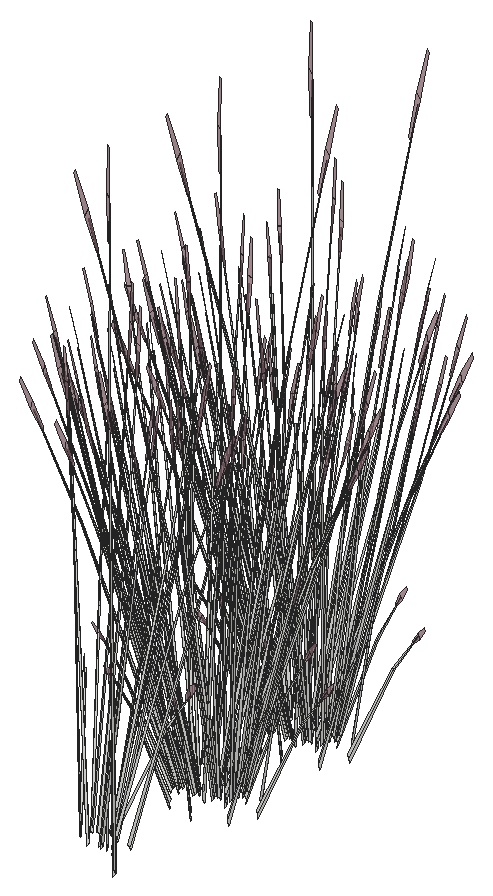
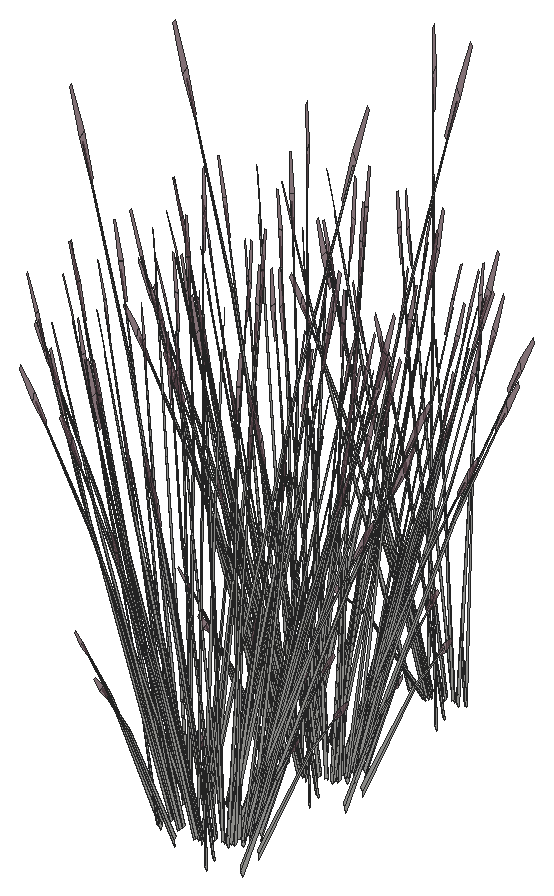
# SketchUp Ruby script. Lengths in inches.
U = 1.inch
M = Sketchup.active_model
def pt(a) = Geom::Point3d.new(a.map { |v| v * U })
def face(e, loops, mat)
  f = e.add_face(loops[0].map { |a| pt(a) })
  loops[1..].each { |l| e.add_face(l.map { |a| pt(a) }).erase! }
  f.material = f.back_material = mat if mat
  f
end
# faces: each face lists its corners as indices into pts; further lists are holes
def faces(e, pts, list, mat = nil) = list.each { |f| face(e, (f[0].is_a?(Array) ? f : [f]).map { |l| l.map { |i| pts[i] } }, mat) }
# xy, xz, yz: faces in a plane at the given z, y or x. An outline is a flat list of corners, or four numbers for a rectangle; further outlines are holes
def ring(l) = l.size == 4 ? [[l[0], l[1]], [l[2], l[1]], [l[2], l[3]], [l[0], l[3]]] : l.each_slice(2).to_a
def flat(e, list, mat, &to3) = list.each { |f| face(e, (f[0].is_a?(Array) ? f : [f]).map { |l| ring(l).map { |u, v| to3.(u, v) } }, mat) }
def xy(e, z, list, mat = nil) = flat(e, list, mat) { |x, y| [x, y, z] }
def xz(e, y, list, mat = nil) = flat(e, list, mat) { |x, z| [x, y, z] }
def yz(e, x, list, mat = nil) = flat(e, list, mat) { |y, z| [x, y, z] }
def lines(e, pts, list) = list.each { |a, b| e.add_line(pt(pts[a]), pt(pts[b])) }
# prism: a flat outline (further loops are holes) pulled along v
def prism(e, loops, v, mat = nil)
  f = face(e, loops, mat); d = Geom::Vector3d.new(v.map { |x| x * U })
  f.pushpull(f.normal.samedirection?(d) ? d.length : -d.length)
end
def box(e, o, s, mat = nil) = prism(e, [[o, [o[0] + s[0], o[1], o[2]], [o[0] + s[0], o[1] + s[1], o[2]], [o[0], o[1] + s[1], o[2]]]], [0, 0, s[2]], mat)
def at(x, y, z, deg = 0) = Geom::Transformation.translation(pt([x, y, z])) * Geom::Transformation.rotation(ORIGIN, Z_AXIS, deg.degrees)
def axes(o, x, y, z) = Geom::Transformation.new([*x, 0, *y, 0, *z, 0, *pt(o).to_a, 1])
def part(name) = M.definitions.add(name)
# library, detail: a bought-in or finely detailed component or shape, given as its bounding box
def library(name, o, s) = part(name).tap { |d| box(d.entities, o, s) }
def detail(e, o, s) = box(e.add_group.entities, o, s)
def put(e, d, t, mat = nil) = e.add_instance(d, t).tap { |i| i.material = mat if mat }
def group(e, t, mat = nil) = e.add_group.tap { |g| g.transformation = t; g.material = mat if mat }.entities
root = M.entities
M.materials.add("LightPink_Translucent").color = [144, 107, 117]
M.materials["LightPink_Translucent"].alpha = 0.75
c1 = part("blade")
p = [[2.15,0.21,22],[0,0.17,0],[0.09,0.45,0],[2.18,0.31,22],[2.29,0.31,22],[0.38,0.45,0],
  [2.48,0.24,33],[2.49,0.24,33],[2.48,0.22,33]]
faces(c1.entities,p,[[0,1,2,3],[4,5,2,3],[6,3,4,7],[8,0,3,6]])
c2 = part("seeds")
p = [[0.3,-0.1,1.38],[-0.01,-0.03,1.59],[-0.01,-0.03,0.03],[0.14,-0.07,-0.07],[0.29,-0.03,3],[0.15,0.01,3.11]]
faces(c2.entities,p,[[0,1,2,3],[1,0,4,5]],"LightPink_Translucent")
c3 = part("blade with seeds")
put(c3.entities,c1,at(0,0,0))
put(c3.entities,c2,axes([2.4,0.25,30.99],[1.5799,-0.05474,1.17369],[-0.12525,1.92788,0.29478],[-0.07173,-0.02425,1.56792]))
put(root,c3,axes([331.86,478.88,52.14],[0.12971,0.3568,-0.45151],[-0.49122,0.06241,-0.34973],[-0.14077,0.09583,0.86392]))
put(root,c3,axes([334.74,478.15,50.51],[-0.01379,-0.36791,1.24828],[0.62424,0.09537,0.52853],[-0.14764,0.20132,1.17828]))
put(root,c3,axes([334.79,479.57,52.14],[0.49824,-0.09289,-0.45151],[0.08716,0.35177,-0.34973],[0.13382,0.10081,0.86392]))
put(root,c3,axes([332.16,478.82,51.43],[0.09401,-0.13431,1.51428],[0.3944,0.27795,0.12244],[-0.17792,0.17323,0.64734]))
put(root,c3,axes([332.27,479.58,52],[-0.34164,0.20573,-0.31292],[-0.3234,-0.23491,0.40398],[-0.04921,0.11936,0.77298]))
put(root,c3,axes([331.09,479.52,52.17],[-0.01255,0.07733,1.54581],[0.35618,0.269,-0.24447],[-0.09325,0.12721,0.12397]))
put(root,c3,axes([333.25,479.75,52.45],[0.49409,-0.18193,-0.10745],[0.24281,0.32289,-0.59638],[0.06519,0.13607,0.90619]))
put(root,c3,axes([332.48,480.38,50.44],[-0.01307,-0.23234,1.01491],[0.32652,0.16572,0.74569],[-0.06422,0.11074,0.22354]))
put(root,c3,axes([332.61,479.48,52.42],[0.36145,0.26255,-0.50118],[-0.38183,0.22994,-0.3882],[-0.055,0.1334,0.95895]))
put(root,c3,axes([333.68,479.74,52.14],[0.49634,0.09796,-0.45151],[-0.17013,0.33585,-0.34973],[0.04551,0.13522,0.86392]))
put(root,c3,axes([333.96,479.04,51.43],[-0.11542,-0.12546,1.51428],[0.53333,-0.10562,0.12244],[0.12054,0.19696,0.64734]))
put(root,c3,axes([333.45,479.94,52],[-0.15222,0.30049,-0.31292],[-0.44409,-0.08764,0.40398],[0.04072,0.12098,0.77298]))
put(root,c3,axes([332.49,479.36,52.72],[-0.01314,0.36145,-0.69681],[-0.55324,-0.02428,0.08409],[-0.05838,0.15313,0.9857]))
put(root,c3,axes([333.02,479.11,51.43],[-0.01236,-0.14998,1.51428],[0.53562,0.09949,0.12244],[-0.03313,0.21373,0.64734]))
put(root,c3,axes([333.5,479.67,52.4],[0.24099,0.31773,-0.62776],[-0.49607,0.17707,0.07576],[0.05635,0.15352,0.88802]))
put(root,c3,axes([333.14,480.48,52.17],[0.064,0.06292,1.54581],[0.51651,0.02472,-0.24447],[0.05194,0.13877,0.12397]))
put(root,c3,axes([332.31,479.87,50.97],[0.01109,-0.20172,1.3638],[0.49896,0.10655,0.18846],[-0.04323,0.21498,0.64398]))
put(root,c3,axes([332.69,487.29,51.43],[0.11542,0.12546,1.51428],[-0.53333,0.10562,0.12244],[-0.12054,-0.19696,0.64734]))
put(root,c3,axes([334.11,487.38,52.4],[-0.24099,-0.31773,-0.62776],[0.49607,-0.17707,0.07576],[-0.05635,-0.15352,0.88802]))
put(root,c3,axes([335.12,487.69,52.4],[0.01314,-0.36145,-0.62776],[0.55324,0.02428,0.07576],[0.05838,-0.15313,0.88802]))
put(root,c3,axes([334.16,487.11,52],[0.15222,-0.30049,-0.31292],[0.44409,0.08764,0.40398],[-0.04072,-0.12098,0.77298]))
put(root,c3,axes([334.5,487.51,51.43],[-0.09401,0.13431,1.51428],[-0.3944,-0.27795,0.12244],[0.17792,-0.17323,0.64734]))
put(root,c3,axes([333.93,487.32,52.14],[-0.49634,-0.09796,-0.45151],[0.17013,-0.33585,-0.34973],[-0.04551,-0.13522,0.86392]))
put(root,c3,axes([334.24,486.48,50.44],[0.06477,0.22786,1.01491],[-0.35932,-0.1262,0.74569],[0.03867,-0.11667,0.22354]))
put(root,c3,axes([335.01,487.57,52.14],[-0.36145,-0.26255,-0.45151],[0.38183,-0.22994,-0.34973],[0.055,-0.1334,0.86392]))
put(root,c3,axes([334.36,487.3,52.45],[-0.49409,0.18193,-0.10745],[-0.24281,-0.32289,-0.59638],[-0.06519,-0.13607,0.90619]))
put(root,c3,axes([335.38,487.71,52.45],[-0.55492,-0.01936,-0.10745],[0.01517,-0.36657,-0.59638],[0.03855,-0.14118,0.90619]))
put(root,c3,axes([335.35,487.47,52],[0.34164,-0.20573,-0.31292],[0.3234,0.23491,0.40398],[0.04921,-0.11936,0.77298]))
put(root,c3,axes([332.39,486.75,50.44],[0.26338,0.136,1.01491],[-0.38358,0.08175,0.74569],[-0.08207,-0.10452,0.22354]))
put(root,c3,axes([333.03,487.47,52.4],[-0.43054,-0.18887,-0.62776],[0.30598,-0.33097,0.07576],[-0.15599,-0.11277,0.88802]))
put(root,c3,axes([332.88,487.22,52],[-0.07798,-0.31474,-0.31292],[0.44579,-0.08311,0.40398],[-0.11974,-0.09019,0.77298]))
put(root,c3,axes([331.92,487.68,51.43],[0.18755,0.06732,1.51428],[-0.38813,0.28243,0.12244],[-0.24191,-0.12741,0.64734]))
put(root,c3,axes([332.83,487.48,52.14],[-0.49824,0.09289,-0.45151],[-0.08716,-0.35177,-0.34973],[-0.13382,-0.10081,0.86392]))
put(root,c3,axes([335.77,488.32,52.4],[0.26374,-0.30832,-0.62776],[0.46217,0.21911,0.07576],[0.15748,-0.11171,0.88802]))
put(root,c3,axes([335.76,488.18,52.14],[-0.12971,-0.3568,-0.45151],[0.49122,-0.06241,-0.34973],[0.14077,-0.09583,0.86392]))
put(root,c3,axes([335.99,488.43,52.45],[-0.46706,-0.21546,-0.10745],[0.26908,-0.31203,-0.59638],[0.13196,-0.10846,0.90619]))
put(root,c3,axes([334.06,489.61,50.9375],[0.43633,0.15757,1.33654],[-0.42745,0.33945,0.52853],[-0.19146,-0.20119,1.12046]))
put(root,c3,axes([336.36,487.47,50.44],[-0.16818,0.19891,1.01491],[-0.14456,-0.26725,0.74569],[0.1389,-0.06697,0.22354]))
put(root,c3,axes([336.12,488.21,52],[0.43951,-0.05584,-0.31292],[0.11606,0.31924,0.40398],[0.12595,-0.08575,0.77298]))
put(root,c3,axes([331.85,487.77,52],[-0.28729,-0.24465,-0.31292],[0.32804,-0.23159,0.40398],[-0.16667,-0.03524,0.77298]))
put(root,c3,axes([332.15,487.9375,52.4],[-0.50473,-0.00941,-0.62776],[0.0339,-0.39618,0.07576],[-0.21383,-0.04181,0.88802]))
put(root,c3,axes([331.98,488.02,52.14],[-0.36663,0.25884,-0.45151],[-0.32109,-0.27343,-0.34973],[-0.18628,-0.03938,0.86392]))
put(root,c3,axes([331.16,488.36,50.44],[0.32236,-0.02796,1.01491],[-0.20448,0.24636,0.74569],[-0.1593,-0.03696,0.22354]))
put(root,c3,axes([332.18,487.75,52.45],[-0.02704,0.39739,-0.10745],[-0.51189,-0.01086,-0.59638],[-0.19715,-0.0276,0.90619]))
put(root,c3,axes([336.01,489.27,52.45],[-0.25405,-0.35383,-0.10745],[0.45089,-0.17388,-0.59638],[0.19001,-0.04668,0.90619]))
put(root,c3,axes([335.98,488.97,52.14],[0.13679,-0.35544,-0.45151],[0.46898,0.12183,-0.34973],[0.18882,-0.03259,0.86392]))
put(root,c3,axes([331.52,488.29,51.43],[0.20943,-0.00885,1.51428],[-0.13893,0.38357,0.12244],[-0.29846,-0.02372,0.64734]))
put(root,c3,axes([335.9,489.1,52.4],[0.44368,-0.17257,-0.62776],[0.24726,0.35524,0.07576],[0.21437,-0.04035,0.88802]))
put(root,c3,axes([336.27,489.13,52],[0.41962,0.10901,-0.31292],[-0.12239,0.31802,0.40398],[0.16894,-0.02916,0.77298]))
put(root,c3,axes([331.34,488.625,52],[-0.41962,-0.10901,-0.31292],[0.12239,-0.31802,0.40398],[-0.16894,0.02916,0.77298]))
put(root,c3,axes([335.13,488.74,51.43],[-0.20943,0.00885,1.51428],[0.13893,-0.38357,0.12244],[0.29846,0.02372,0.64734]))
put(root,c3,axes([332.62,488.57,50.95],[0.14352,-0.05653,1.56454],[0.04949,0.39467,0.12244],[-0.31087,0.05237,0.55918]))
put(root,c3,axes([337.16,489.19,50.44],[-0.31197,0.06451,1.01491],[0.14684,-0.26661,0.74569],[0.1655,0.01824,0.22354]))
put(root,c3,axes([331.63,488.79,52.14],[-0.13679,0.35544,-0.45151],[-0.46898,-0.12183,-0.34973],[-0.18882,0.03259,0.86392]))
put(root,c3,axes([331.61,488.48,52.45],[0.25405,0.35383,-0.10745],[-0.45089,0.17388,-0.59638],[-0.19001,0.04668,0.90619]))
put(root,c3,axes([336.62,490.02,51.47],[-0.09664,-0.32847,-0.03085],[0.45676,-0.07551,-0.13989],[0.09538,0.02082,0.4614]))
put(root,c3,axes([335.4375,490.01,52.45],[0.02704,-0.39739,-0.10745],[0.51189,0.01086,-0.59638],[0.19715,0.0276,0.90619]))
put(root,c3,axes([331.61,488.97,51.43],[0.17519,-0.08265,1.51428],[0.14749,0.38193,0.12244],[-0.27504,0.08632,0.64734]))
put(root,c3,axes([335.46,489.82,52.4],[0.50473,0.00941,-0.62776],[-0.0339,0.39618,0.07576],[0.21383,0.04181,0.88802]))
put(root,c3,axes([330.7,490.31,50.44],[0.21042,-0.1771,1.01491],[0.08303,0.28036,0.74569],[-0.15207,0.0502,0.22354]))
put(root,c3,axes([335.77,489.98,52],[0.28729,0.24465,-0.31292],[-0.32804,0.23159,0.40398],[0.16667,0.03524,0.77298]))
put(root,c3,axes([331.49,489.54,52],[-0.43951,0.05584,-0.31292],[-0.11606,-0.31924,0.40398],[-0.12595,0.08575,0.77298]))
put(root,c3,axes([334.73,489.35,51.43],[-0.18755,-0.06732,1.51428],[0.38813,-0.28243,0.12244],[0.24191,0.12741,0.64734]))
put(root,c3,axes([334.77,488.47,51.95],[-0.4363,-0.20303,1.22187],[0.46069,-0.31611,0.5272],[0.14077,0.1905,1.18105]))
put(root,c3,axes([331.625,489.32,52.45],[0.46706,0.21546,-0.10745],[-0.26908,0.31203,-0.59638],[-0.13196,0.10846,0.90619]))
put(root,c3,axes([335.43,490.12,50.44],[-0.28429,-0.11236,1.01491],[0.36709,-0.11416,0.74569],[0.09901,0.0967,0.22354]))
put(root,c3,axes([334.43,490.4375,52.45],[0.30087,-0.33447,-0.10745],[0.43572,0.19269,-0.59638],[0.15146,0.0945,0.90619]))
put(root,c3,axes([332.25,489.23,51.43],[0.12611,-0.12006,1.51428],[0.31843,0.32408,0.12244],[-0.2184,0.14759,0.64734]))
put(root,c3,axes([331.86,489.58,52.14],[0.12971,0.3568,-0.45151],[-0.49122,0.06241,-0.34973],[-0.14077,0.09583,0.86392]))
put(root,c3,axes([334.74,488.85,50.51],[-0.01379,-0.36791,1.24828],[0.62424,0.09537,0.52853],[-0.14764,0.20132,1.17828]))
put(root,c3,axes([334.79,490.27,52.14],[0.49824,-0.09289,-0.45151],[0.08716,0.35177,-0.34973],[0.13382,0.10081,0.86392]))
put(root,c3,axes([332.16,489.52,51.43],[0.09401,-0.13431,1.51428],[0.3944,0.27795,0.12244],[-0.17792,0.17323,0.64734]))
put(root,c3,axes([332.27,490.28,52],[-0.34164,0.20573,-0.31292],[-0.3234,-0.23491,0.40398],[-0.04921,0.11936,0.77298]))
put(root,c3,axes([332.69,496.06,51.43],[0.11542,0.12546,1.51428],[-0.53333,0.10562,0.12244],[-0.12054,-0.19696,0.64734]))
put(root,c3,axes([333.25,490.45,52.45],[0.49409,-0.18193,-0.10745],[0.24281,0.32289,-0.59638],[0.06519,0.13607,0.90619]))
put(root,c3,axes([332.48,491.08,50.44],[-0.01307,-0.23234,1.01491],[0.32652,0.16572,0.74569],[-0.06422,0.11074,0.22354]))
put(root,c3,axes([334.11,496.16,52.4],[-0.24099,-0.31773,-0.62776],[0.49607,-0.17707,0.07576],[-0.05635,-0.15352,0.88802]))
put(root,c3,axes([332.61,490.18,52.42],[0.36145,0.26255,-0.50118],[-0.38183,0.22994,-0.3882],[-0.055,0.1334,0.95895]))
put(root,c3,axes([333.68,490.4375,52.14],[0.49634,0.09796,-0.45151],[-0.17013,0.33585,-0.34973],[0.04551,0.13522,0.86392]))
put(root,c3,axes([333.96,489.74,51.43],[-0.11542,-0.12546,1.51428],[0.53333,-0.10562,0.12244],[0.12054,0.19696,0.64734]))
put(root,c3,axes([335.12,496.47,52.4],[0.01314,-0.36145,-0.62776],[0.55324,0.02428,0.07576],[0.05838,-0.15313,0.88802]))
put(root,c3,axes([333.45,490.64,52],[-0.15222,0.30049,-0.31292],[-0.44409,-0.08764,0.40398],[0.04072,0.12098,0.77298]))
put(root,c3,axes([334.16,495.89,52],[0.15222,-0.30049,-0.31292],[0.44409,0.08764,0.40398],[-0.04072,-0.12098,0.77298]))
put(root,c3,axes([334.5,496.29,51.43],[-0.09401,0.13431,1.51428],[-0.3944,-0.27795,0.12244],[0.17792,-0.17323,0.64734]))
put(root,c3,axes([332.49,490.0625,52.72],[-0.01314,0.36145,-0.69681],[-0.55324,-0.02428,0.08409],[-0.05838,0.15313,0.9857]))
put(root,c3,axes([333.93,496.09,52.14],[-0.49634,-0.09796,-0.45151],[0.17013,-0.33585,-0.34973],[-0.04551,-0.13522,0.86392]))
put(root,c3,axes([334.24,495.25,50.44],[0.06477,0.22786,1.01491],[-0.35932,-0.1262,0.74569],[0.03867,-0.11667,0.22354]))
put(root,c3,axes([333.02,489.81,51.43],[-0.01236,-0.14998,1.51428],[0.53562,0.09949,0.12244],[-0.03313,0.21373,0.64734]))
put(root,c3,axes([335.01,496.35,52.14],[-0.36145,-0.26255,-0.45151],[0.38183,-0.22994,-0.34973],[0.055,-0.1334,0.86392]))
put(root,c3,axes([333.5,490.375,52.4],[0.24099,0.31773,-0.62776],[-0.49607,0.17707,0.07576],[0.05635,0.15352,0.88802]))
put(root,c3,axes([334.36,496.08,52.45],[-0.49409,0.18193,-0.10745],[-0.24281,-0.32289,-0.59638],[-0.06519,-0.13607,0.90619]))
put(root,c3,axes([335.38,496.49,52.45],[-0.55492,-0.01936,-0.10745],[0.01517,-0.36657,-0.59638],[0.03855,-0.14118,0.90619]))
put(root,c3,axes([335.35,496.25,52],[0.34164,-0.20573,-0.31292],[0.3234,0.23491,0.40398],[0.04921,-0.11936,0.77298]))
put(root,c3,axes([332.39,495.53,50.44],[0.26338,0.136,1.01491],[-0.38358,0.08175,0.74569],[-0.08207,-0.10452,0.22354]))
put(root,c3,axes([333.03,496.25,52.4],[-0.43054,-0.18887,-0.62776],[0.30598,-0.33097,0.07576],[-0.15599,-0.11277,0.88802]))
put(root,c3,axes([332.88,496,52],[-0.07798,-0.31474,-0.31292],[0.44579,-0.08311,0.40398],[-0.11974,-0.09019,0.77298]))
put(root,c3,axes([332.31,490.57,50.97],[0.01109,-0.20172,1.3638],[0.49896,0.10655,0.18846],[-0.04323,0.21498,0.64398]))
put(root,c3,axes([331.92,496.46,51.43],[0.18755,0.06732,1.51428],[-0.38813,0.28243,0.12244],[-0.24191,-0.12741,0.64734]))
put(root,c3,axes([332.83,496.26,52.14],[-0.49824,0.09289,-0.45151],[-0.08716,-0.35177,-0.34973],[-0.13382,-0.10081,0.86392]))
put(root,c3,axes([335.77,497.1,52.4],[0.26374,-0.30832,-0.62776],[0.46217,0.21911,0.07576],[0.15748,-0.11171,0.88802]))
put(root,c3,axes([335.76,496.95,52.14],[-0.12971,-0.3568,-0.45151],[0.49122,-0.06241,-0.34973],[0.14077,-0.09583,0.86392]))
put(root,c3,axes([335.99,497.21,52.45],[-0.46706,-0.21546,-0.10745],[0.26908,-0.31203,-0.59638],[0.13196,-0.10846,0.90619]))
put(root,c3,axes([334.06,498.39,50.9375],[0.43633,0.15757,1.33654],[-0.42745,0.33945,0.52853],[-0.19146,-0.20119,1.12046]))
put(root,c3,axes([336.36,496.24,50.44],[-0.16818,0.19891,1.01491],[-0.14456,-0.26725,0.74569],[0.1389,-0.06697,0.22354]))
put(root,c3,axes([336.12,496.99,52],[0.43951,-0.05584,-0.31292],[0.11606,0.31924,0.40398],[0.12595,-0.08575,0.77298]))
put(root,c3,axes([331.85,496.55,52],[-0.28729,-0.24465,-0.31292],[0.32804,-0.23159,0.40398],[-0.16667,-0.03524,0.77298]))
put(root,c3,axes([332.15,496.72,52.4],[-0.50473,-0.00941,-0.62776],[0.0339,-0.39618,0.07576],[-0.21383,-0.04181,0.88802]))
put(root,c3,axes([331.98,496.8,52.14],[-0.36663,0.25884,-0.45151],[-0.32109,-0.27343,-0.34973],[-0.18628,-0.03938,0.86392]))
put(root,c3,axes([331.16,497.14,50.44],[0.32236,-0.02796,1.01491],[-0.20448,0.24636,0.74569],[-0.1593,-0.03696,0.22354]))
put(root,c3,axes([332.18,496.52,52.45],[-0.02704,0.39739,-0.10745],[-0.51189,-0.01086,-0.59638],[-0.19715,-0.0276,0.90619]))
put(root,c3,axes([336.01,498.05,52.45],[-0.25405,-0.35383,-0.10745],[0.45089,-0.17388,-0.59638],[0.19001,-0.04668,0.90619]))
put(root,c3,axes([335.98,497.75,52.14],[0.13679,-0.35544,-0.45151],[0.46898,0.12183,-0.34973],[0.18882,-0.03259,0.86392]))
put(root,c3,axes([331.52,497.07,51.43],[0.20943,-0.00885,1.51428],[-0.13893,0.38357,0.12244],[-0.29846,-0.02372,0.64734]))
put(root,c3,axes([335.9,497.875,52.4],[0.44368,-0.17257,-0.62776],[0.24726,0.35524,0.07576],[0.21437,-0.04035,0.88802]))
put(root,c3,axes([336.27,497.91,52],[0.41962,0.10901,-0.31292],[-0.12239,0.31802,0.40398],[0.16894,-0.02916,0.77298]))
put(root,c3,axes([331.34,497.4,52],[-0.41962,-0.10901,-0.31292],[0.12239,-0.31802,0.40398],[-0.16894,0.02916,0.77298]))
put(root,c3,axes([335.13,497.51,51.43],[-0.20943,0.00885,1.51428],[0.13893,-0.38357,0.12244],[0.29846,0.02372,0.64734]))
put(root,c3,axes([332.62,497.35,50.95],[0.14352,-0.05653,1.56454],[0.04949,0.39467,0.12244],[-0.31087,0.05237,0.55918]))
put(root,c3,axes([337.16,497.97,50.44],[-0.31197,0.06451,1.01491],[0.14684,-0.26661,0.74569],[0.1655,0.01824,0.22354]))
put(root,c3,axes([331.63,497.5625,52.14],[-0.13679,0.35544,-0.45151],[-0.46898,-0.12183,-0.34973],[-0.18882,0.03259,0.86392]))
put(root,c3,axes([331.61,497.26,52.45],[0.25405,0.35383,-0.10745],[-0.45089,0.17388,-0.59638],[-0.19001,0.04668,0.90619]))
put(root,c3,axes([336.62,498.79,51.47],[-0.09664,-0.32847,-0.03085],[0.45676,-0.07551,-0.13989],[0.09538,0.02082,0.4614]))
put(root,c3,axes([335.4375,498.78,52.45],[0.02704,-0.39739,-0.10745],[0.51189,0.01086,-0.59638],[0.19715,0.0276,0.90619]))
put(root,c3,axes([331.61,497.75,51.43],[0.17519,-0.08265,1.51428],[0.14749,0.38193,0.12244],[-0.27504,0.08632,0.64734]))
put(root,c3,axes([335.46,498.59,52.4],[0.50473,0.00941,-0.62776],[-0.0339,0.39618,0.07576],[0.21383,0.04181,0.88802]))
put(root,c3,axes([330.7,499.08,50.44],[0.21042,-0.1771,1.01491],[0.08303,0.28036,0.74569],[-0.15207,0.0502,0.22354]))
put(root,c3,axes([335.77,498.76,52],[0.28729,0.24465,-0.31292],[-0.32804,0.23159,0.40398],[0.16667,0.03524,0.77298]))
put(root,c3,axes([331.49,498.32,52],[-0.43951,0.05584,-0.31292],[-0.11606,-0.31924,0.40398],[-0.12595,0.08575,0.77298]))
put(root,c3,axes([334.73,498.13,51.43],[-0.18755,-0.06732,1.51428],[0.38813,-0.28243,0.12244],[0.24191,0.12741,0.64734]))
put(root,c3,axes([334.77,497.24,51.95],[-0.4363,-0.20303,1.22187],[0.46069,-0.31611,0.5272],[0.14077,0.1905,1.18105]))
put(root,c3,axes([331.625,498.1,52.45],[0.46706,0.21546,-0.10745],[-0.26908,0.31203,-0.59638],[-0.13196,0.10846,0.90619]))
put(root,c3,axes([335.43,498.9,50.44],[-0.28429,-0.11236,1.01491],[0.36709,-0.11416,0.74569],[0.09901,0.0967,0.22354]))
put(root,c3,axes([334.43,499.22,52.45],[0.30087,-0.33447,-0.10745],[0.43572,0.19269,-0.59638],[0.15146,0.0945,0.90619]))
put(root,c3,axes([332.25,498,51.43],[0.12611,-0.12006,1.51428],[0.31843,0.32408,0.12244],[-0.2184,0.14759,0.64734]))
put(root,c3,axes([331.86,498.36,52.14],[0.12971,0.3568,-0.45151],[-0.49122,0.06241,-0.34973],[-0.14077,0.09583,0.86392]))
put(root,c3,axes([334.74,497.63,50.51],[-0.01379,-0.36791,1.24828],[0.62424,0.09537,0.52853],[-0.14764,0.20132,1.17828]))
put(root,c3,axes([334.79,499.05,52.14],[0.49824,-0.09289,-0.45151],[0.08716,0.35177,-0.34973],[0.13382,0.10081,0.86392]))
put(root,c3,axes([332.16,498.3,51.43],[0.09401,-0.13431,1.51428],[0.3944,0.27795,0.12244],[-0.17792,0.17323,0.64734]))
put(root,c3,axes([332.27,499.06,52],[-0.34164,0.20573,-0.31292],[-0.3234,-0.23491,0.40398],[-0.04921,0.11936,0.77298]))
put(root,c3,axes([333.25,499.23,52.45],[0.49409,-0.18193,-0.10745],[0.24281,0.32289,-0.59638],[0.06519,0.13607,0.90619]))
put(root,c3,axes([332.48,499.86,50.44],[-0.01307,-0.23234,1.01491],[0.32652,0.16572,0.74569],[-0.06422,0.11074,0.22354]))
put(root,c3,axes([332.61,498.96,52.42],[0.36145,0.26255,-0.50118],[-0.38183,0.22994,-0.3882],[-0.055,0.1334,0.95895]))
put(root,c3,axes([333.68,499.21,52.14],[0.49634,0.09796,-0.45151],[-0.17013,0.33585,-0.34973],[0.04551,0.13522,0.86392]))
put(root,c3,axes([333.96,498.52,51.43],[-0.11542,-0.12546,1.51428],[0.53333,-0.10562,0.12244],[0.12054,0.19696,0.64734]))
put(root,c3,axes([333.45,499.42,52],[-0.15222,0.30049,-0.31292],[-0.44409,-0.08764,0.40398],[0.04072,0.12098,0.77298]))
put(root,c3,axes([332.49,498.84,52.72],[-0.01314,0.36145,-0.69681],[-0.55324,-0.02428,0.08409],[-0.05838,0.15313,0.9857]))
put(root,c3,axes([333.02,498.58,51.43],[-0.01236,-0.14998,1.51428],[0.53562,0.09949,0.12244],[-0.03313,0.21373,0.64734]))
put(root,c3,axes([333.5,499.15,52.4],[0.24099,0.31773,-0.62776],[-0.49607,0.17707,0.07576],[0.05635,0.15352,0.88802]))
put(root,c3,axes([332.31,499.35,50.97],[0.01109,-0.20172,1.3638],[0.49896,0.10655,0.18846],[-0.04323,0.21498,0.64398]))
